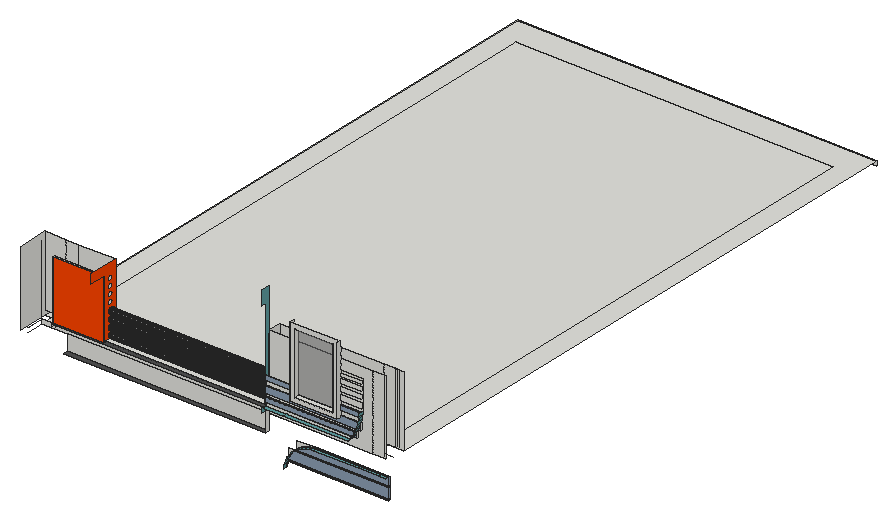
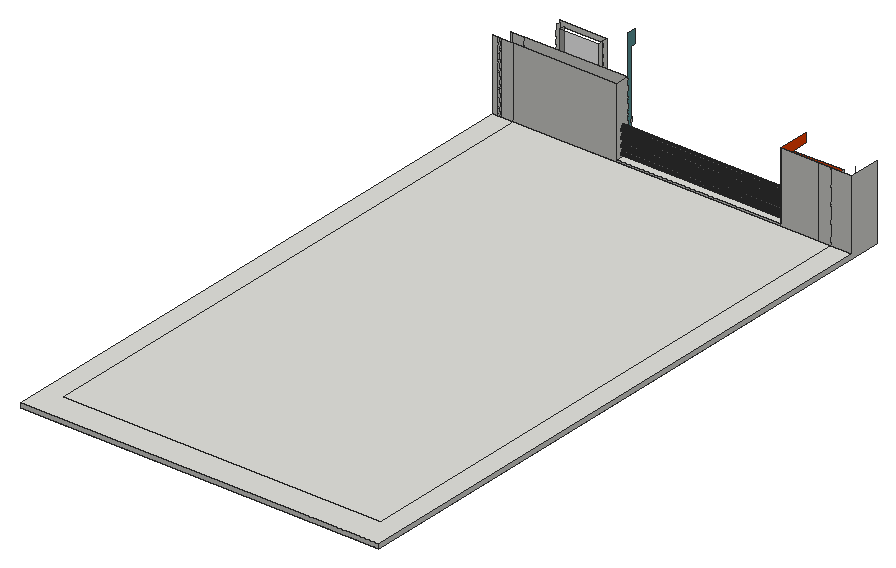
# SketchUp Ruby script. Lengths in inches.
U = 1.inch
M = Sketchup.active_model
def pt(a) = Geom::Point3d.new(a.map { |v| v * U })
def face(e, loops, mat)
  f = e.add_face(loops[0].map { |a| pt(a) })
  loops[1..].each { |l| e.add_face(l.map { |a| pt(a) }).erase! }
  f.material = f.back_material = mat if mat
  f
end
# faces: each face lists its corners as indices into pts; further lists are holes
def faces(e, pts, list, mat = nil) = list.each { |f| face(e, (f[0].is_a?(Array) ? f : [f]).map { |l| l.map { |i| pts[i] } }, mat) }
# xy, xz, yz: faces in a plane at the given z, y or x. An outline is a flat list of corners, or four numbers for a rectangle; further outlines are holes
def ring(l) = l.size == 4 ? [[l[0], l[1]], [l[2], l[1]], [l[2], l[3]], [l[0], l[3]]] : l.each_slice(2).to_a
def flat(e, list, mat, &to3) = list.each { |f| face(e, (f[0].is_a?(Array) ? f : [f]).map { |l| ring(l).map { |u, v| to3.(u, v) } }, mat) }
def xy(e, z, list, mat = nil) = flat(e, list, mat) { |x, y| [x, y, z] }
def xz(e, y, list, mat = nil) = flat(e, list, mat) { |x, z| [x, y, z] }
def yz(e, x, list, mat = nil) = flat(e, list, mat) { |y, z| [x, y, z] }
def lines(e, pts, list) = list.each { |a, b| e.add_line(pt(pts[a]), pt(pts[b])) }
# prism: a flat outline (further loops are holes) pulled along v
def prism(e, loops, v, mat = nil)
  f = face(e, loops, mat); d = Geom::Vector3d.new(v.map { |x| x * U })
  f.pushpull(f.normal.samedirection?(d) ? d.length : -d.length)
end
def box(e, o, s, mat = nil) = prism(e, [[o, [o[0] + s[0], o[1], o[2]], [o[0] + s[0], o[1] + s[1], o[2]], [o[0], o[1] + s[1], o[2]]]], [0, 0, s[2]], mat)
def at(x, y, z, deg = 0) = Geom::Transformation.translation(pt([x, y, z])) * Geom::Transformation.rotation(ORIGIN, Z_AXIS, deg.degrees)
def axes(o, x, y, z) = Geom::Transformation.new([*x, 0, *y, 0, *z, 0, *pt(o).to_a, 1])
def part(name) = M.definitions.add(name)
# library, detail: a bought-in or finely detailed component or shape, given as its bounding box
def library(name, o, s) = part(name).tap { |d| box(d.entities, o, s) }
def detail(e, o, s) = box(e.add_group.entities, o, s)
def put(e, d, t, mat = nil) = e.add_instance(d, t).tap { |i| i.material = mat if mat }
def group(e, t, mat = nil) = e.add_group.tap { |g| g.transformation = t; g.material = mat if mat }.entities
root = M.entities
M.materials.add("[0024_OrangeRed]").color = [255, 69, 0]
M.materials.add("[0081_CadetBlue]").color = [95, 158, 160]
M.materials.add("[0110_LightSlateGray]").color = [139, 158, 178]
M.materials.add("[0133_Gray]").color = [128, 128, 128]
M.materials.add("[0135_DarkGray]").color = [81, 81, 81]
M.materials.add("[Translucent Glass Gray]").color = [128, 128, 128]
M.materials["[Translucent Glass Gray]"].alpha = 0.5
xy(root,341.1,[[176.04,8,245.1875,9]],"[0110_LightSlateGray]")
xy(root,342.19,[[176.41,8,245.1875,9]],"[0110_LightSlateGray]")
xy(root,348.6875,[[180.67,8,245.1875,9]],"[0110_LightSlateGray]")
xy(root,349.97,[[182.03,8,245.1875,9]],"[0110_LightSlateGray]")
xy(root,352.5,[[22.75,9,160.53,12]],"[0135_DarkGray]")
xy(root,355.26,[[195.95,8,226.59,9],[226.59,8,245.1875,9]])
xy(root,355.26,[[195.95,6,226.59,8],[226.59,6,240.375,8],[240.375,6,245.1875,8]],"[0081_CadetBlue]")
xy(root,363,[[5,12,14,21],[14,12,231.375,79.875],[0,21,5,79.875],[5,21,14,79.875],[0,79.875,5,85.875],
  [5,79.875,14,85.875],[14,79.875,231.375,85.875],[0,85.875,5,405.4375],[5,85.875,14,405.4375],[14,85.875,231.375,405.4375],
  [0,405.4375,5,414.4375],[5,405.4375,14,405.4375,14,424.625,0,424.625,0,414.4375,5,414.4375],[14,405.4375,231.375,424.625]])
xy(root,366,[[0,21,14,21,14,405.4375,231.375,405.4375,231.375,21,245.1875,21,245.1875,424.625,0,424.625],[14,21,231.375,405.4375]])
xy(root,367.625,[[14,10.4375,48.4375,12],[48.4375,12,160.53,21]])
xy(root,367.625,[[14,9,160.53,9,160.53,12,48.4375,12,48.4375,10.4375,14,10.4375]],"[0135_DarkGray]")
xy(root,368.91,[[160.53,6,174.8,9],[174.8,6,218.8125,9]],"[0081_CadetBlue]")
xy(root,371.68,[[221.11,8,223.55,9]])
xy(root,371.68,[[160.53,8,221.11,9]],"[0110_LightSlateGray]")
xy(root,374.99,[[160.53,8,223.55,9]],"[0110_LightSlateGray]")
xy(root,377.14,[[224.22,8,226.15,9]])
xy(root,377.14,[[160.53,8,224.22,9]],"[0110_LightSlateGray]")
xy(root,379.97,[[179.47,6,211.78,8],[179.47,8,211.78,9]])
xy(root,381.46,[[211.78,8,226.15,9]],"[0110_LightSlateGray]")
xy(root,381.77,[[160.53,8,179.47,9]],"[0110_LightSlateGray]")
xy(root,383.03,[[182.53,6,208.72,9]])
xy(root,384.77,[[211.78,8,225.89,9]],"[0110_LightSlateGray]")
xy(root,385.08,[[160.53,8,179.47,9]],"[0110_LightSlateGray]")
xz(root,6,[[[179.47,379.97,211.78,428.35],[182.53,383.03,208.72,425.29]]])
xz(root,8,[[176.41,342.19,245.1875,342.19,245.1875,348.6875,180.67,348.6875,179.17,346.98,177.63,344.68],[182.03,349.97,245.1875,349.97,245.1875,355.26,195.95,355.26,193.19,355.08,190.48,354.54,187.86,353.65,185.375,352.42,183.07,350.88],[160.53,371.68,223.55,374.99],[160.53,377.14,226.15,377.14,226.15,381.46,211.78,381.46,211.78,379.97,179.47,379.97,179.47,381.77,160.53,381.77],[211.78,384.77,225.89,388.02],
  [160.53,385.08,179.47,388.02]],"[0110_LightSlateGray]")
xz(root,9,[[176.04,341.1,245.1875,341.1,245.1875,342.19,176.41,342.19],[176.41,342.19,177.63,344.68,179.17,346.98,180.67,348.6875,176.41,348.6875],[176.41,342.19,177.63,344.68,179.17,346.98,180.67,348.6875,245.1875,348.6875,245.1875,342.19],[180.67,348.6875,245.1875,348.6875,245.1875,349.97,182.03,349.97,180.99,349.06],[182.03,349.97,183.07,350.88,185.375,352.42,187.86,353.65,190.48,354.54,193.19,355.08,195.95,355.26,182.03,355.26],
  [182.03,349.97,183.07,350.88,185.375,352.42,187.86,353.65,190.48,354.54,193.19,355.08,195.95,355.26,245.1875,355.26,245.1875,349.97],[160.53,368.91,218.8125,368.91,220.01,370.26,221.11,371.68,160.53,371.68],[160.53,371.68,221.05,374.99],[221.05,371.68,221.11,371.68,222.125,373.17,223.04,374.72,223.18,374.99,221.05,374.99],[221.11,371.68,222.125,373.17,223.04,374.72,223.18,374.99,223.55,374.99,223.55,371.68],
  [160.53,374.99,223.18,374.99,223.86,376.32,224.22,377.14,160.53,377.14],[160.53,377.14,160.53,381.77,179.47,381.77,179.47,379.97,211.78,379.97,211.78,381.46,224.22,381.46,224.22,377.14],[224.22,377.14,224.57,377.97,225.1875,379.66,225.6875,381.39,225.7,381.46,224.22,381.46],[224.22,377.14,224.57,377.97,225.1875,379.66,225.6875,381.39,225.7,381.46,226.15,381.46,226.15,377.14],[211.78,381.46,225.7,381.46,226.08,383.15,226.36,384.93,226.53,386.72,226.59,388.52,226.59,408.61,211.78,408.61,211.78,407.32,226.5625,407.32,226.5625,404.77,211.78,404.77,211.78,403.8125,226.5625,403.8125,226.5625,400.39,211.78,400.39,211.78,399.05,226.5625,399.05,226.5625,395.43,211.78,395.43,211.78,393.9,226.5625,393.9,226.5625,389.79,211.78,389.79,211.78,388.02,225.89,388.02,225.89,384.77,211.78,384.77],
  [160.53,381.77,179.47,385.08],[211.78,384.77,225.89,388.02],[160.53,385.08,179.47,388.02]])
xz(root,9,[[182.53,383.03,208.72,425.29]],"[Translucent Glass Gray]")
xz(root,10.4375,[[14,367.625,48.4375,407.79]],"[0024_OrangeRed]")
xz(root,12,[[22.75,352.5,160.53,363],[5,363,14,366],[14,363,160.53,367.625],[160.53,363,231.375,414],[231.375,363,238.75,414],
  [238.75,363,240.375,366],[238.75,366,240.375,414],[14,367.625,48.4375,407.79]])
xz(root,21,[[0,366,14,414],[14,366,22.75,414],[22.75,366,22.75,414,48.4375,414,48.4375,367.625,160.53,367.625,160.53,366],[160.53,366,231.375,414],[231.375,366,238.75,414],
  [238.75,366,240.375,414],[240.375,366,241.9375,414],[241.9375,366,245.1875,414]])
xz(root,424.625,[[0,363,245.1875,366]])
yz(root,0,[[0,363,0,414,21,414,21,366,424.625,366,424.625,363]])
yz(root,14,[[9,366,12,367.625],[10.4375,367.625,12,407.79]])
yz(root,48.4375,[[[12,367.625,21,367.625,21,414,0,414,0,407.79,12,407.79],[16.15,373.09,15.65,373.16,15.18,373.35,14.78,373.66,14.48,374.0625,14.28,374.53,14.22,375.03,14.28,375.53,14.48,376,14.78,376.4,15.18,376.71,15.65,376.9,16.15,376.97,16.65,376.9,17.12,376.71,17.52,376.4,17.83,376,18.02,375.53,18.09,375.03,18.02,374.53,17.83,374.0625,17.52,373.66,17.12,373.35,16.65,373.16],[16.15,378.09,15.65,378.16,15.18,378.35,14.78,378.66,14.48,379.0625,14.28,379.53,14.22,380.03,14.28,380.53,14.48,381,14.78,381.4,15.18,381.71,15.65,381.9,16.15,381.97,16.65,381.9,17.12,381.71,17.52,381.4,17.83,381,18.02,380.53,18.09,380.03,18.02,379.53,17.83,379.0625,17.52,378.66,17.12,378.35,16.65,378.16],[16.15,383.03,15.65,383.1,15.18,383.29,14.78,383.6,14.48,384,14.28,384.47,14.22,384.97,14.28,385.47,14.48,385.9375,14.78,386.34,15.18,386.65,15.65,386.84,16.15,386.91,16.65,386.84,17.12,386.65,17.52,386.34,17.83,385.9375,18.02,385.47,18.09,384.97,18.02,384.47,17.83,384,17.52,383.6,17.12,383.29,16.65,383.1],[16.15,387.97,15.65,388.04,15.18,388.23,14.78,388.54,14.48,388.9375,14.28,389.41,14.22,389.91,14.28,390.41,14.48,390.875,14.78,391.28,15.18,391.59,15.65,391.78,16.15,391.84,16.65,391.78,17.12,391.59,17.52,391.28,17.83,390.875,18.02,390.41,18.09,389.91,18.02,389.41,17.83,388.9375,17.52,388.54,17.12,388.23,16.65,388.04],[16.15,392.91,15.65,392.97,15.18,393.17,14.78,393.47,14.48,393.875,14.28,394.34,14.22,394.84,14.28,395.35,14.48,395.8125,14.78,396.21,15.18,396.52,15.65,396.72,16.15,396.78,16.65,396.72,17.12,396.52,17.52,396.21,17.83,395.8125,18.02,395.35,18.09,394.84,18.02,394.34,17.83,393.875,17.52,393.47,17.12,393.17,16.65,392.97],[16.15,397.84,15.65,397.91,15.18,398.1,14.78,398.41,14.48,398.8125,14.28,399.28,14.22,399.78,14.28,400.28,14.48,400.75,14.78,401.15,15.18,401.46,15.65,401.65,16.15,401.72,16.65,401.65,17.12,401.46,17.52,401.15,17.83,400.75,18.02,400.28,18.09,399.78,18.02,399.28,17.83,398.8125,17.52,398.41,17.12,398.1,16.65,397.91],[16.15,402.78,15.65,402.85,15.18,403.04,14.78,403.35,14.48,403.75,14.28,404.22,14.22,404.72,14.28,405.22,14.48,405.6875,14.78,406.09,15.18,406.4,15.65,406.59,16.15,406.66,16.65,406.59,17.12,406.4,17.52,406.09,17.83,405.6875,18.02,405.22,18.09,404.72,18.02,404.22,17.83,403.75,17.52,403.35,17.12,403.04,16.65,402.85],[16.15,368.28,15.65,368.35,15.18,368.54,14.78,368.85,14.48,369.25,14.28,369.72,14.22,370.22,14.28,370.72,14.48,371.1875,14.78,371.59,15.18,371.9,15.65,372.09,16.15,372.16,16.65,372.09,17.12,371.9,17.52,371.59,17.83,371.1875,18.02,370.72,18.09,370.22,18.02,369.72,17.83,369.25,17.52,368.85,17.12,368.54,16.65,368.35]],[10.4375,367.625,12,407.79]],"[0024_OrangeRed]")
yz(root,160.5,[[16.15,373.09,16.65,373.16,17.12,373.35,17.52,373.66,17.83,374.0625,18.02,374.53,18.09,375.03,18.02,375.53,17.83,376,17.52,376.4,17.12,376.71,16.65,376.9,16.15,376.97,15.65,376.9,15.18,376.71,14.78,376.4,14.47,376,14.28,375.53,14.22,375.03,14.28,374.53,14.47,374.0625,14.78,373.66,15.18,373.35,15.65,373.16]])
yz(root,160.53,[[9,352.5,12,366],[9,366,12,367.625],[12,367.625,21,414],[16.15,368.28,16.65,368.35,17.12,368.54,17.52,368.85,17.83,369.25,18.02,369.72,18.09,370.22,18.02,370.72,17.83,371.1875,17.52,371.59,17.12,371.9,16.65,372.09,16.15,372.16,15.65,372.09,15.18,371.9,14.78,371.59,14.47,371.1875,14.28,370.72,14.22,370.22,14.28,369.72,14.47,369.25,14.78,368.85,15.18,368.54,15.65,368.35],[8,371.68,9,374.99],
  [8,377.14,9,381.77],[16.15,378.09,16.65,378.16,17.12,378.35,17.52,378.66,17.83,379.0625,18.02,379.53,18.09,380.03,18.02,380.53,17.83,381,17.52,381.4,17.12,381.71,16.65,381.9,16.15,381.97,15.65,381.9,15.18,381.71,14.78,381.4,14.47,381,14.28,380.53,14.22,380.03,14.28,379.53,14.47,379.0625,14.78,378.66,15.18,378.35,15.65,378.16],[16.15,383.03,16.65,383.1,17.12,383.29,17.52,383.6,17.83,384,18.02,384.47,18.09,384.97,18.02,385.47,17.83,385.9375,17.52,386.34,17.12,386.65,16.65,386.84,16.15,386.91,15.65,386.84,15.18,386.65,14.78,386.34,14.47,385.9375,14.28,385.47,14.22,384.97,14.28,384.47,14.47,384,14.78,383.6,15.18,383.29,15.65,383.1],[8,385.08,9,388.02]])
yz(root,160.53,[[6,366,6,368.91,9,368.91,9,431.57,6,431.57,6,441.0625,12,441.0625,12,367.625,9,367.625,9,366]],"[0081_CadetBlue]")
yz(root,179.47,[[6,379.97,6,428.35,9,428.35,9,426.8,8,426.8,8,423.16,9,423.16,9,420.17,8,420.17,8,417.42,9,417.42,9,415.15,8,415.15,8,412.46,9,412.46,9,411.25,8,411.25,8,408.61,9,408.61,9,407.32,8,407.32,8,404.77,9,404.77,9,403.8125,8,403.8125,8,400.39,9,400.39,9,399.05,8,399.05,8,395.43,9,395.43,9,393.9,8,393.9,8,389.79,9,389.79,9,388.02,8,388.02,8,385.08,9,385.08,9,381.77,8,381.77,8,379.97],[8,379.97,9,381.77],[8,385.08,9,388.02]])
yz(root,182.53,[[6,383.03,9,425.29]])
yz(root,208.72,[[6,383.03,9,425.29]])
yz(root,211.78,[[6,379.97,8,379.97,8,381.46,9,381.46,9,384.77,8,384.77,8,388.02,9,388.02,9,389.79,8,389.79,8,393.9,9,393.9,9,395.43,8,395.43,8,399.05,9,399.05,9,400.39,8,400.39,8,403.8125,9,403.8125,9,404.77,8,404.77,8,407.32,9,407.32,9,408.61,8,408.61,8,411.25,9,411.25,9,412.46,8,412.46,8,415.15,9,415.15,9,417.42,8,417.42,8,420.17,9,420.17,9,423.16,8,423.16,8,426.8,6,426.8],[8,379.97,9,381.46],[8,384.77,9,388.02]])
yz(root,223.55,[[8,371.68,9,374.99]])
yz(root,225.89,[[8,384.77,9,388.02]])
yz(root,226.15,[[8,377.14,9,381.46]])
yz(root,245.1875,[[8,342.19,9,348.6875],[8,349.97,9,355.26]],"[0110_LightSlateGray]")
p = [[174.98,6,336.86],[174.98,8,336.86],[175.52,8,339.57],[175.52,6,339.57],[174.98,9,336.86],[175.52,9,339.57],
  [176.04,8,341.1],[176.04,9,341.1],[176.41,9,342.19],[176.41,8,342.19],[176.41,6,342.19],[177.63,8,344.68],
  [177.63,6,344.68],[177.63,9,344.68],[179.17,8,346.98],[179.17,6,346.98],[179.17,9,346.98],[180.67,8,348.6875],
  [180.67,9,348.6875],[180.99,9,349.06],[180.99,6,349.06],[182.03,9,349.97],[182.03,8,349.97],[183.07,8,350.88],
  [183.07,6,350.88],[183.07,9,350.88],[185.375,8,352.42],[185.375,6,352.42],[185.375,9,352.42],[187.86,8,353.65],
  [187.86,6,353.65],[187.86,9,353.65],[190.48,8,354.54],[190.48,6,354.54],[190.48,9,354.54],[193.19,8,355.08],
  [193.19,6,355.08],[193.19,9,355.08],[195.95,8,355.26],[195.95,6,355.26],[195.95,9,355.26],[48.4375,15.18,368.54],
  [48.4375,15.65,368.35],[160.53,15.65,368.35],[160.53,15.18,368.54],[48.4375,16.15,368.28],[160.53,16.15,368.28],[48.4375,16.65,368.35],
  [160.53,16.65,368.35],[48.4375,17.12,368.54],[160.53,17.12,368.54],[48.4375,14.78,368.85],[160.53,14.78,368.85],[48.4375,17.52,368.85],
  [160.53,17.52,368.85],[48.4375,14.48,369.25],[160.53,14.47,369.25],[48.4375,17.83,369.25],[160.53,17.83,369.25],[220.01,9,370.26],
  [218.8125,9,368.91],[218.8125,6,368.91],[220.01,6,370.26],[48.4375,14.28,369.72],[160.53,14.28,369.72],[48.4375,18.02,369.72],
  [160.53,18.02,369.72],[48.4375,14.22,370.22],[160.53,14.22,370.22],[48.4375,18.09,370.22],[160.53,18.09,370.22],[48.4375,14.28,370.72],
  [160.53,14.28,370.72],[48.4375,18.02,370.72],[160.53,18.02,370.72],[221.11,9,371.68],[221.11,6,371.68],[221.11,8,371.68],
  [48.4375,14.48,371.1875],[160.53,14.47,371.1875],[48.4375,17.83,371.1875],[160.53,17.83,371.1875],[48.4375,14.78,371.59],[160.53,14.78,371.59],
  [48.4375,17.52,371.59],[160.53,17.52,371.59],[48.4375,15.18,371.9],[160.53,15.18,371.9],[48.4375,17.12,371.9],[160.53,17.12,371.9],
  [222.125,9,373.17],[222.125,6,373.17],[48.4375,15.65,372.09],[160.53,15.65,372.09],[48.4375,16.65,372.09],[160.53,16.65,372.09],
  [48.4375,16.15,372.16],[160.53,16.15,372.16],[48.4375,15.65,373.16],[48.4375,16.15,373.09],[160.5,16.15,373.09],[160.5,15.65,373.16],
  [48.4375,16.65,373.16],[160.5,16.65,373.16],[223.04,9,374.72],[223.04,6,374.72],[48.4375,15.18,373.35],[160.5,15.18,373.35],
  [48.4375,17.12,373.35],[160.5,17.12,373.35],[48.4375,14.78,373.66],[160.5,14.78,373.66],[48.4375,17.52,373.66],[160.5,17.52,373.66],
  [48.4375,14.48,374.0625],[160.5,14.47,374.0625],[48.4375,17.83,374.0625],[160.5,17.83,374.0625],[48.4375,14.28,374.53],[160.5,14.28,374.53],
  [48.4375,18.02,374.53],[160.5,18.02,374.53],[48.4375,14.22,375.03],[160.5,14.22,375.03],[48.4375,18.09,375.03],[160.5,18.09,375.03],
  [223.86,9,376.32],[223.18,9,374.99],[223.86,6,376.32],[48.4375,14.28,375.53],[160.5,14.28,375.53],[48.4375,18.02,375.53],
  [160.5,18.02,375.53],[48.4375,14.48,376],[160.5,14.47,376],[48.4375,17.83,376],[160.5,17.83,376],[48.4375,14.78,376.4],
  [160.5,14.78,376.4],[48.4375,17.52,376.4],[160.5,17.52,376.4],[224.57,9,377.97],[224.22,9,377.14],[224.57,6,377.97],
  [48.4375,15.18,376.71],[160.5,15.18,376.71],[48.4375,17.12,376.71],[160.5,17.12,376.71],[48.4375,15.65,376.9],[160.5,15.65,376.9],
  [48.4375,16.65,376.9],[160.5,16.65,376.9],[48.4375,16.15,376.97],[160.5,16.15,376.97],[225.1875,9,379.66],[225.1875,6,379.66],
  [48.4375,15.65,378.16],[48.4375,16.15,378.09],[160.53,16.15,378.09],[160.53,15.65,378.16],[48.4375,16.65,378.16],[160.53,16.65,378.16],
  [48.4375,15.18,378.35],[160.53,15.18,378.35],[48.4375,17.12,378.35],[160.53,17.12,378.35],[48.4375,14.78,378.66],[160.53,14.78,378.66],
  [48.4375,17.52,378.66],[160.53,17.52,378.66],[48.4375,14.48,379.0625],[160.53,14.47,379.0625],[48.4375,17.83,379.0625],[160.53,17.83,379.0625],
  [48.4375,14.28,379.53],[160.53,14.28,379.53],[48.4375,18.02,379.53],[160.53,18.02,379.53],[48.4375,14.22,380.03],[160.53,14.22,380.03],
  [48.4375,18.09,380.03],[160.53,18.09,380.03],[225.6875,9,381.39],[225.6875,6,381.39],[48.4375,14.28,380.53],[160.53,14.28,380.53],
  [48.4375,18.02,380.53],[160.53,18.02,380.53],[48.4375,14.48,381],[160.53,14.47,381],[48.4375,17.83,381],[160.53,17.83,381],
  [48.4375,14.78,381.4],[160.53,14.78,381.4],[48.4375,17.52,381.4],[160.53,17.52,381.4],[226.08,9,383.15],[225.7,9,381.46],
  [226.08,6,383.15],[48.4375,15.18,381.71],[160.53,15.18,381.71],[48.4375,17.12,381.71],[160.53,17.12,381.71],[48.4375,15.65,381.9],
  [160.53,15.65,381.9],[48.4375,16.65,381.9],[160.53,16.65,381.9],[48.4375,16.15,381.97],[160.53,16.15,381.97],[48.4375,15.65,383.1],
  [48.4375,16.15,383.03],[160.53,16.15,383.03],[160.53,15.65,383.1],[48.4375,16.65,383.1],[160.53,16.65,383.1],[226.36,9,384.93],
  [226.36,6,384.93],[48.4375,15.18,383.29],[160.53,15.18,383.29],[48.4375,17.12,383.29],[160.53,17.12,383.29],[48.4375,14.78,383.6],
  [160.53,14.78,383.6],[48.4375,17.52,383.6],[160.53,17.52,383.6],[48.4375,14.48,384],[160.53,14.47,384],[48.4375,17.83,384],
  [160.53,17.83,384],[48.4375,14.28,384.47],[160.53,14.28,384.47],[48.4375,18.02,384.47],[160.53,18.02,384.47],[48.4375,14.22,384.97],
  [160.53,14.22,384.97],[48.4375,18.09,384.97],[160.53,18.09,384.97],[226.53,9,386.72],[226.53,6,386.72],[48.4375,14.28,385.47],
  [160.53,14.28,385.47],[48.4375,18.02,385.47],[160.53,18.02,385.47],[48.4375,14.48,385.9375],[160.53,14.47,385.9375],[48.4375,17.83,385.9375],
  [160.53,17.83,385.9375],[48.4375,14.78,386.34],[160.53,14.78,386.34],[48.4375,17.52,386.34],[160.53,17.52,386.34],[48.4375,15.18,386.65],
  [160.53,15.18,386.65],[48.4375,17.12,386.65],[160.53,17.12,386.65],[48.4375,15.65,386.84],[160.53,15.65,386.84],[48.4375,16.65,386.84],
  [160.53,16.65,386.84],[226.59,9,388.52],[226.59,6,388.52],[48.4375,16.15,386.91],[160.53,16.15,386.91],[231.375,405.4375,363],
  [240.375,405.4375,363],[240.375,12,366],[245.1875,12,366],[5,12,363],[5,0,363],[5,12,366],
  [5,0,366],[5,12,414]]
faces(root,p,[[0,1,2,3],[3,2,6,7,8,9,10],[10,9,11,12],[12,11,14,15],[15,14,17,18,19,20],[19,21,22,23,24,20],[24,23,26,27],[27,26,29,30],
  [30,29,32,33],[33,32,35,36],[36,35,38,39],[59,60,61,62],[75,59,62,76,77],[90,75,77,76,91],[104,90,91,105],[126,127,104,105,128],
  [141,142,126,128,143],[154,141,143,155],[182,154,155,183],[196,197,182,183,198],[215,196,198,216],[237,215,216,238],[259,237,238,260]],"[0081_CadetBlue]")
faces(root,p,[[4,5,2,1],[5,7,6,2],[8,13,11,9],[13,16,14,11],[16,18,17,14],[21,25,23,22],[25,28,26,23],[28,31,29,26],
  [31,34,32,29],[34,37,35,32],[37,40,38,35]])
faces(root,p,[[41,42,43,44],[42,45,46,43],[45,47,48,46],[47,49,50,48],[51,41,44,52],[49,53,54,50],[55,51,52,56],[53,57,58,54],
  [63,55,56,64],[57,65,66,58],[67,63,64,68],[65,69,70,66],[71,67,68,72],[69,73,74,70],[78,71,72,79],[73,80,81,74],
  [82,78,79,83],[80,84,85,81],[86,82,83,87],[84,88,89,85],[92,86,87,93],[88,94,95,89],[96,92,93,97],[94,96,97,95],
  [98,99,100,101],[99,102,103,100],[106,98,101,107],[102,108,109,103],[110,106,107,111],[108,112,113,109],[114,110,111,115],[112,116,117,113],
  [118,114,115,119],[116,120,121,117],[122,118,119,123],[120,124,125,121],[129,122,123,130],[124,131,132,125],[133,129,130,134],[131,135,136,132],
  [137,133,134,138],[135,139,140,136],[144,137,138,145],[139,146,147,140],[148,144,145,149],[146,150,151,147],[152,148,149,153],[150,152,153,151],
  [156,157,158,159],[157,160,161,158],[162,156,159,163],[160,164,165,161],[166,162,163,167],[164,168,169,165],[170,166,167,171],[168,172,173,169],
  [174,170,171,175],[172,176,177,173],[178,174,175,179],[176,180,181,177],[184,178,179,185],[180,186,187,181],[188,184,185,189],[186,190,191,187],
  [192,188,189,193],[190,194,195,191],[199,192,193,200],[194,201,202,195],[203,199,200,204],[201,205,206,202],[207,203,204,208],[205,207,208,206],
  [209,210,211,212],[210,213,214,211],[217,209,212,218],[213,219,220,214],[221,217,218,222],[219,223,224,220],[225,221,222,226],[223,227,228,224],
  [229,225,226,230],[227,231,232,228],[233,229,230,234],[231,235,236,232],[239,233,234,240],[235,241,242,236],[243,239,240,244],[241,245,246,242],
  [247,243,244,248],[245,249,250,246],[251,247,248,252],[249,253,254,250],[255,251,252,256],[253,257,258,254],[261,255,256,262],[257,261,262,258]],"[0133_Gray]")
lines(root,p,[[263,264],[265,266],[267,268],[269,270],[269,271]])
